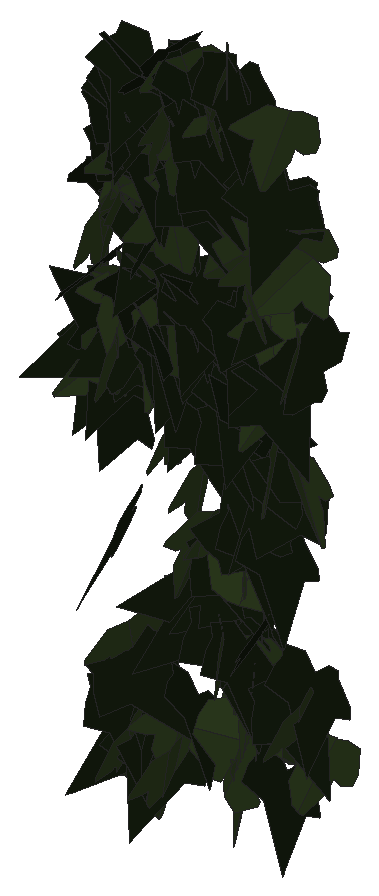
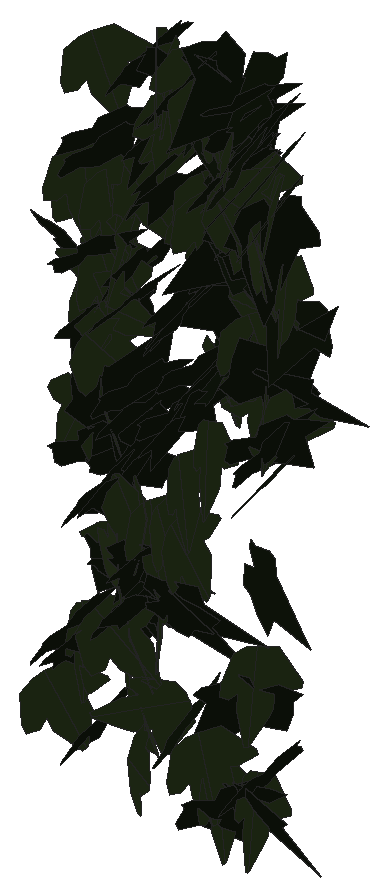
# SketchUp Ruby script. Lengths in inches.
U = 1.inch
M = Sketchup.active_model
def pt(a) = Geom::Point3d.new(a.map { |v| v * U })
def face(e, loops, mat)
  f = e.add_face(loops[0].map { |a| pt(a) })
  loops[1..].each { |l| e.add_face(l.map { |a| pt(a) }).erase! }
  f.material = f.back_material = mat if mat
  f
end
# faces: each face lists its corners as indices into pts; further lists are holes
def faces(e, pts, list, mat = nil) = list.each { |f| face(e, (f[0].is_a?(Array) ? f : [f]).map { |l| l.map { |i| pts[i] } }, mat) }
# xy, xz, yz: faces in a plane at the given z, y or x. An outline is a flat list of corners, or four numbers for a rectangle; further outlines are holes
def ring(l) = l.size == 4 ? [[l[0], l[1]], [l[2], l[1]], [l[2], l[3]], [l[0], l[3]]] : l.each_slice(2).to_a
def flat(e, list, mat, &to3) = list.each { |f| face(e, (f[0].is_a?(Array) ? f : [f]).map { |l| ring(l).map { |u, v| to3.(u, v) } }, mat) }
def xy(e, z, list, mat = nil) = flat(e, list, mat) { |x, y| [x, y, z] }
def xz(e, y, list, mat = nil) = flat(e, list, mat) { |x, z| [x, y, z] }
def yz(e, x, list, mat = nil) = flat(e, list, mat) { |y, z| [x, y, z] }
def lines(e, pts, list) = list.each { |a, b| e.add_line(pt(pts[a]), pt(pts[b])) }
# prism: a flat outline (further loops are holes) pulled along v
def prism(e, loops, v, mat = nil)
  f = face(e, loops, mat); d = Geom::Vector3d.new(v.map { |x| x * U })
  f.pushpull(f.normal.samedirection?(d) ? d.length : -d.length)
end
def box(e, o, s, mat = nil) = prism(e, [[o, [o[0] + s[0], o[1], o[2]], [o[0] + s[0], o[1] + s[1], o[2]], [o[0], o[1] + s[1], o[2]]]], [0, 0, s[2]], mat)
def at(x, y, z, deg = 0) = Geom::Transformation.translation(pt([x, y, z])) * Geom::Transformation.rotation(ORIGIN, Z_AXIS, deg.degrees)
def axes(o, x, y, z) = Geom::Transformation.new([*x, 0, *y, 0, *z, 0, *pt(o).to_a, 1])
def part(name) = M.definitions.add(name)
# library, detail: a bought-in or finely detailed component or shape, given as its bounding box
def library(name, o, s) = part(name).tap { |d| box(d.entities, o, s) }
def detail(e, o, s) = box(e.add_group.entities, o, s)
def put(e, d, t, mat = nil) = e.add_instance(d, t).tap { |i| i.material = mat if mat }
def group(e, t, mat = nil) = e.add_group.tap { |g| g.transformation = t; g.material = mat if mat }.entities
root = M.entities
M.materials.add("efeu1").color = [18, 25, 13]
M.materials.add("efeu2").color = [43, 57, 29]
c1 = part("ivyleaf_9")
p = [[1.54,2.16,1.25],[1.36,2.04,1.19],[-0.21,0.99,0.68],[-0.71,1.11,0.82],[-0.85,0.86,0.67],[-0.8,0.17,0.21],
  [-0.9,-0.01,0.1],[-0.67,-0.16,-0.02],[-0.08,-0.08,-0.05],[-0.03,-0.6,-0.4],[0.65,-0.88,-0.66],[0.83,-0.6,-0.49],
  [1.29,-0.42,-0.43],[1.8125,-0.07,-0.26],[1.21,0.44,0.15]]
faces(c1.entities,p,[[0,1,2,3,4,5,6,7,8,9,10,11,12,13,14]],"efeu1")
c2 = part("ivyleaf_10")
p = [[0,0.5,-0.03],[-0.0625,2.02,-0.43],[-0.19,2.01,-0.46],[-0.54,1.05,-0.29],[-0.52,0.625,-0.18],[-0.83,0.76,-0.28],
  [-1.16,0.64,-0.33],[-1.15,0.33,-0.24],[-0.77,-0.39,0.02],[-0.3,-0.51,0.16],[0.04,-0.48,0.23],[-0.02,2.01,-0.4375],
  [-0.06,2.01,-0.43],[0.04,-0.49,0.23],[0.67,-0.49,0.14],[1.38,0.36,-0.2],[1.375,0.51,-0.24],[0.81,0.65,-0.19],
  [0.62,0.59,-0.15],[0.6,1.09,-0.28],[0.5,1.23,-0.31]]
faces(c2.entities,p,[[0,1,2,3,4,5,6,7,8,9,10],[11,12,0,13,14,15,16,17,18,19,20]],"efeu2")
put(root,c1,axes([15.86,223.1875,230.26],[0.24677,0.30074,-0.3141],[-0.1921,-0.24861,-0.38896],[-0.39013,0.31264,-0.00716]))
put(root,c1,axes([15.21,223.49,229.13],[-0.44051,-0.07875,0.22305],[-0.21292,-0.07339,-0.44641],[0.10305,-0.48827,0.03112]))
put(root,c2,axes([17.25,223.3,223.22],[0.3938,-0.27521,-0.13851],[0.11664,-0.07489,0.4804],[-0.28517,-0.41067,0.00522]))
put(root,c1,axes([17.35,223.44,225.26],[0.03816,-0.49443,-0.06386],[-0.01235,0.06309,-0.49585],[0.49839,0.03942,-0.0074]))
put(root,c2,axes([17.53,223.3125,231.32],[-0.30315,-0.07469,0.39054],[-0.37436,-0.11188,-0.31199],[0.13399,-0.48157,0.01191]))
put(root,c2,axes([17.13,223.14,225.3125],[0.25962,-0.35479,-0.23817],[-0.02245,0.26697,-0.42217],[0.42672,0.2299,0.12269]))
put(root,c1,axes([15.59,223.49,232.23],[0.11472,-0.48546,0.03423],[0.00403,-0.03422,-0.49881],[0.48664,0.11473,-0.00394]))
put(root,c1,axes([17.7,223.23,226.99],[-0.45124,-0.18685,0.10709],[0.11532,0.00032,0.48652],[-0.18188,0.46378,0.0428]))
put(root,c2,axes([15.62,223.3,232.11],[-0.28032,-0.41388,0.01113],[-0.00701,-0.0087,-0.49988],[0.41397,-0.28041,-0.00092]))
put(root,c2,axes([15.84,223.23,230.14],[0.04541,0.05609,-0.49476],[-0.48178,0.13048,-0.02942],[0.12581,0.4794,0.0659]))
put(root,c1,axes([17.85,223.28,225.91],[-0.26617,0.38506,-0.17573],[0.10204,-0.14309,-0.4681],[-0.41078,-0.28505,-0.00241]))
put(root,c2,axes([15.21,223.46,231.27],[0.24763,-0.41301,0.13453],[0.05903,-0.12142,-0.48143],[0.43034,0.25432,-0.01137]))
put(root,c2,axes([17.3,223.51,224.67],[0.31176,-0.23758,0.31042],[0.24588,-0.18948,-0.39197],[0.30389,0.39705,-0.00131]))
put(root,c1,axes([18.74,223.23,229.96],[-0.3068,0.24738,0.3077],[-0.28197,0.13547,-0.39005],[-0.27635,-0.41286,0.05638]))
put(root,c2,axes([14.95,223.625,228.75],[0.10418,0.16205,-0.46139],[-0.21361,-0.40928,-0.19198],[-0.4399,0.23712,-0.01604]))
put(root,c1,axes([16.83,223.35,232.36],[0.12613,-0.43747,-0.20666],[-0.01007,0.21114,-0.45312],[0.48373,0.11847,0.04445]))
put(root,c2,axes([16.16,223.43,231.67],[-0.31513,-0.34515,0.17768],[-0.10555,-0.14404,-0.46702],[0.37357,-0.33185,0.01792]))
put(root,c1,axes([15.26,223.67,232.83],[-0.01589,-0.45199,0.21319],[-0.00074,-0.21328,-0.45223],[0.49975,-0.01469,0.00611]))
put(root,c2,axes([16.0625,223.44,232.81],[0.11558,-0.48244,0.06237],[0.00528,-0.06286,-0.496],[0.48643,0.11532,-0.00944]))
put(root,c1,axes([16.43,223.7,229.87],[-0.06282,-0.44757,0.21386],[0.01955,-0.21763,-0.44973],[0.49565,-0.04814,0.04484]))
put(root,c1,axes([15.47,223.64,232.97],[-0.16707,-0.46805,0.05495],[-0.00932,-0.05501,-0.49688],[0.47117,-0.16705,0.00966]))
put(root,c2,axes([18.2,223.35,229.95],[0.26547,-0.4145,-0.08784],[-0.00901,0.09811,-0.4902],[0.42361,0.26185,0.04463]))
put(root,c1,axes([17.79,223.59,226.87],[0.05152,-0.49494,0.04876],[-0.00165,-0.04919,-0.49757],[0.49734,0.05111,-0.0067]))
put(root,c2,axes([18.29,223.3,224.55],[0.03,-0.47542,-0.1519],[-0.00786,0.15171,-0.47636],[0.49904,0.03097,0.00163]))
put(root,c2,axes([15.48,223.3,224.87],[-0.17216,-0.45368,-0.12057],[0.02813,0.11822,-0.48501],[0.46858,-0.17378,-0.01518]))
put(root,c1,axes([17.84,223.66,232.11],[-0.19505,-0.45699,0.05581],[-0.00161,-0.05994,-0.49639],[0.46039,-0.19382,0.02191]))
put(root,c2,axes([15.37,223.49,229.89],[-0.32684,-0.34111,0.16377],[-0.05059,-0.17506,-0.46561],[0.37499,-0.32093,0.07992]))
put(root,c1,axes([15.02,222.98,230.23],[0.10792,0.42864,0.23371],[-0.03637,0.24575,-0.43392],[-0.48686,0.07665,0.08422]))
put(root,c1,axes([17.84,223.64,223.38],[0.05191,-0.48216,0.12178],[-0.00176,-0.12261,-0.48473],[0.4973,0.04989,-0.01443]))
put(root,c1,axes([15.3,223.51,226.43],[-0.34724,0.20864,-0.29308],[0.22682,-0.18921,-0.40343],[-0.27925,-0.41312,0.03675]))
put(root,c2,axes([17.75,223.42,231.16],[-0.17923,-0.46553,0.03403],[-0.01528,-0.03058,-0.49883],[0.46652,-0.17985,-0.00326]))
put(root,c2,axes([16.66,223.1,232.64],[-0.11534,-0.27013,-0.40463],[0.19892,0.35331,-0.29257],[0.44399,-0.22847,0.02596]))
put(root,c1,axes([15.83,223.41,230.98],[-0.36766,0.30773,-0.14188],[0.0951,-0.10723,-0.47902],[-0.32524,-0.37921,0.02032]))
put(root,c1,axes([17.04,223.51,225.42],[-0.04802,-0.46925,-0.16583],[0.04016,0.1624,-0.47118],[0.49607,-0.05858,0.02209]))
put(root,c1,axes([17.48,223.58,227.08],[0.05363,-0.49662,-0.02218],[-0.00311,0.02197,-0.49951],[0.49711,0.05371,-0.00073]))
put(root,c1,axes([16.58,223.42,232.98],[0.18734,-0.43311,-0.1653],[0.00438,0.17994,-0.46648],[0.46356,0.17333,0.07121]))
put(root,c1,axes([17.29,223.31,230.3],[0.22014,-0.34812,-0.28346],[-0.07722,0.28164,-0.40585],[0.44224,0.22246,0.07024]))
put(root,c2,axes([16.16,223.375,231.28],[-0.33531,-0.36449,-0.06867],[0.07402,0.02496,-0.49386],[0.36344,-0.34136,0.03722]))
put(root,c1,axes([15.51,223.72,233.31],[-0.22317,-0.43975,0.08259],[0.01864,-0.10135,-0.48927],[0.44705,-0.2153,0.06163]))
put(root,c2,axes([15.86,223.49,229.29],[0.46364,-0.18186,0.04437],[0.03985,-0.01991,-0.49801],[0.1829,0.46533,-0.00397]))
put(root,c1,axes([15.78,223.74,230.86],[-0.26233,-0.40787,0.12178],[-0.04372,-0.11647,-0.48428],[0.42341,-0.26472,0.02545]))
put(root,c1,axes([15.5,223.33,224.49],[0.00889,-0.2958,-0.40302],[0.13521,0.38948,-0.28288],[0.48129,-0.10396,0.08691]))
put(root,c1,axes([15.63,223.6,232.18],[0.02676,-0.49747,-0.04252],[0.01403,0.04331,-0.49792],[0.49909,0.02546,0.01627]))
put(root,c2,axes([15.36,223.5,229.1875],[-0.28977,0.20402,-0.35272],[0.28631,-0.20602,-0.35438],[-0.28993,-0.40735,0.00257]))
put(root,c2,axes([15.99,223.42,223.01],[0.00465,-0.49582,-0.06434],[-0.00297,0.06431,-0.49584],[0.49997,0.00499,-0.00235]))
put(root,c1,axes([15.07,223.65,229.21],[0.10962,0.07724,0.48168],[-0.43915,-0.19938,0.13191],[0.21245,-0.45198,0.02413]))
put(root,c2,axes([17.88,223.57,233.21],[-0.31192,-0.35447,0.16448],[-0.04207,-0.17877,-0.46505],[0.3885,-0.30396,0.0817]))
put(root,c1,axes([17.27,223.81,229.78],[-0.12009,-0.43821,0.2087],[0.02981,-0.22124,-0.4474],[0.48445,-0.09502,0.07926]))
put(root,c1,axes([16.68,223.6,225.49],[-0.49621,-0.02764,0.05486],[-0.05466,-0.00502,-0.49698],[0.02803,-0.49921,0.00196]))
put(root,c1,axes([17.75,223.48,229.39],[0.02124,-0.43309,-0.24896],[0.0132,0.24958,-0.43305],[0.49937,0.01183,0.02203]))
put(root,c2,axes([15.19,223.34,228.98],[0.1464,-0.4323,-0.20416],[0.02054,0.21901,-0.44901],[0.47765,0.12308,0.08188]))
put(root,c1,axes([15.63,223.79,229.33],[0.02375,-0.33085,0.37413],[0.13642,-0.35601,-0.32349],[0.48044,0.11745,0.07336]))
put(root,c2,axes([14.88,223.37,230.83],[0.11212,-0.45357,-0.17804],[0.04122,0.19087,-0.46029],[0.48552,0.08853,0.0802]))
put(root,c2,axes([18.15,223.52,231.125],[0.36253,0.14287,-0.31331],[-0.32168,-0.02182,-0.38216],[-0.12287,0.47866,0.0761]))
put(root,c1,axes([16.3,223.75,233.33],[0.02018,-0.49002,0.09731],[0.00339,-0.09725,-0.49044],[0.49958,0.02046,-0.0006]))
put(root,c2,axes([17.82,223.41,229.89],[0.44554,0.21775,0.06389],[-0.05854,-0.02571,0.49589],[0.21925,-0.44936,0.00258]))
put(root,c1,axes([16.27,223.76,223.92],[0.12233,-0.43677,0.21041],[0.06538,-0.20016,-0.4535],[0.48038,0.13846,0.00814]))
put(root,c2,axes([17.39,223.33,226.2],[0.40222,0.25461,-0.15297],[0.12372,0.09048,0.47593],[0.27003,-0.4207,0.00979]))
put(root,c1,axes([15.87,223.75,229.33],[0.07157,-0.48017,0.11964],[0.01452,-0.11879,-0.48547],[0.49464,0.07297,-0.00307]))
put(root,c1,axes([16.42,223.55,231.86],[0.06953,-0.46074,-0.18134],[0.055,0.18917,-0.45955],[0.49208,0.04395,0.07699]))
put(root,c2,axes([16.93,223.22,233.22],[-0.22253,0.26397,0.36166],[-0.25815,0.25434,-0.34448],[-0.36584,-0.34004,0.02309]))
put(root,c2,axes([16.88,223.34,223.83],[-0.07816,-0.12764,-0.47707],[0.4657,0.14169,-0.11421],[0.16435,-0.4622,0.09674]))
put(root,c1,axes([16.95,223.71,233.54],[0.05308,-0.49677,0.01999],[0.00139,-0.01995,-0.4996],[0.49717,0.0531,-0.00073]))
put(root,c2,axes([16.4,223.69,226.57],[0.03393,-0.46005,0.19287],[0.03089,-0.19101,-0.46104],[0.49789,0.04321,0.01546]))
put(root,c1,axes([16.08,223.8125,229.32],[-0.17918,-0.46,0.07933],[0.01217,-0.08955,-0.49177],[0.46663,-0.1743,0.04329]))
put(root,c2,axes([16.64,223.46,232.72],[-0.28671,-0.3972,-0.10015],[0.09238,0.05639,-0.48814],[0.39908,-0.29841,0.04105]))
put(root,c2,axes([17.68,223.64,230.17],[-0.14365,-0.46264,0.12379],[0.01813,-0.1344,-0.48126],[0.47858,-0.13378,0.05539]))
put(root,c1,axes([14.93,223.88,227.95],[-0.0649,-0.40738,0.28254],[0.04362,-0.28854,-0.40601],[0.49385,-0.02805,0.07299]))
put(root,c1,axes([15.2,223.5,233.45],[0.40522,-0.28286,0.07608],[0.10466,0.01853,-0.48857],[0.27357,0.41188,0.07423]))
put(root,c2,axes([17.06,223.79,223.09],[0.14308,-0.29862,0.37464],[0.25412,-0.28415,-0.32354],[0.40614,0.28299,0.07045]))
put(root,c1,axes([16.48,223.66,233.55],[-0.34415,-0.27309,-0.23871],[0.19262,0.14123,-0.43926],[0.30734,-0.3943,0.008]))
put(root,c2,axes([17.39,223.82,225.82],[0.07444,-0.25911,-0.42109],[0.16703,-0.38762,0.26804],[-0.46536,-0.18058,0.02885]))
put(root,c1,axes([16.26,223.64,232.63],[-0.43972,0.18535,-0.1493],[0.11487,-0.10941,-0.47417],[-0.20844,-0.4513,0.05363]))
put(root,c1,axes([16.61,223.51,232.05],[0.20943,-0.4047,-0.20581],[-0.03505,0.21156,-0.45168],[0.45267,0.20362,0.06025]))
put(root,c1,axes([17.96,223.58,224.62],[0.09813,-0.45117,-0.19189],[0.01714,0.19873,-0.45849],[0.48998,0.08341,0.05447]))
put(root,c2,axes([15.51,223.82,231.92],[-0.12978,-0.2891,0.38675],[-0.11233,-0.37141,-0.31533],[0.46962,-0.16873,0.03146]))
put(root,c1,axes([16,223.57,233.09],[0.35881,-0.34609,-0.03838],[-0.02774,0.02653,-0.49852],[0.34711,0.35988,-0.00017]))
put(root,c1,axes([15.06,223.69,223.61],[0.1087,-0.48477,-0.05638],[-0.0015,0.05743,-0.49669],[0.48804,0.10815,0.01103]))
put(root,c2,axes([16.99,223.77,226.72],[-0.16941,0.22803,-0.41146],[0.18439,-0.37015,-0.28105],[-0.43278,-0.24697,0.04132]))
put(root,c1,axes([17.875,223.86,227.6],[-0.35818,-0.33385,0.10122],[-0.05736,-0.08674,-0.48907],[0.34411,-0.36196,0.02384]))
put(root,c2,axes([15.125,223.36,231.96],[-0.29089,0.34506,0.21522],[-0.14504,0.15918,-0.45125],[-0.37993,-0.32496,0.00749]))
put(root,c2,axes([17.53,223.79,228.23],[0.27149,-0.28888,0.3047],[0.21672,-0.21437,-0.39634],[0.35962,0.34727,0.00881]))
put(root,c2,axes([17.63,223.86,229.07],[-0.18357,-0.31543,0.34177],[-0.0139,-0.36355,-0.34299],[0.46488,-0.13542,0.1247]))
put(root,c2,axes([15.33,223.46,223.16],[-0.00778,-0.45175,-0.21414],[0.00087,0.21416,-0.45181],[0.49994,-0.00741,-0.00255]))
put(root,c1,axes([16.36,223.68,228.39],[0.13404,-0.46899,-0.10992],[-0.00666,0.11229,-0.48718],[0.48165,0.13207,0.02386]))
put(root,c2,axes([18.06,223.61,231.48],[-0.32962,-0.37321,0.04544],[-0.02985,-0.03426,-0.49793],[0.37478,-0.33097,0.00031]))
put(root,c1,axes([15.36,223.76,232.52],[0.25717,-0.40741,0.13371],[0.08257,-0.10595,-0.48162],[0.42077,0.2698,0.01279]))
put(root,c2,axes([15.76,223.62,232.71],[-0.35355,0.31487,-0.1608],[0.08403,-0.14605,-0.47075],[-0.34342,-0.3599,0.05036]))
put(root,c1,axes([15.6875,223.85,223.06],[-0.26929,-0.42114,-0.01092],[0.00374,0.01058,-0.49987],[0.42127,-0.26931,-0.00255]))
put(root,c1,axes([16.99,223.69,228.37],[0.06031,-0.47306,-0.15024],[0.00631,0.15207,-0.47627],[0.49631,0.05555,0.02432]))
put(root,c1,axes([15.34,223.71,223.18],[-0.49579,0.06457,-0.0052],[0.00487,-0.00285,-0.49997],[-0.06459,-0.49581,0.0022]))
put(root,c2,axes([16.67,223.69,226.71],[0.10039,-0.48832,0.03824],[0.00541,-0.03793,-0.49853],[0.48979,0.1005,-0.00234]))
put(root,c1,axes([15.16,223.44,231.73],[0.2273,0.40725,-0.18023],[-0.1021,-0.1493,-0.46614],[-0.43349,0.24871,0.01529]))
put(root,c1,axes([16.26,223.66,230.28],[0.1301,-0.45127,-0.17155],[-0.00733,0.1758,-0.46802],[0.48272,0.12429,0.03913]))
put(root,c2,axes([17.59,223.73,224.93],[-0.28094,-0.20232,0.36075],[-0.30334,-0.19568,-0.34597],[0.28118,-0.41325,-0.01279]))
put(root,c1,axes([15.32,223.71,232.18],[0.21657,-0.44655,-0.06074],[0.00316,0.06889,-0.49522],[0.45065,0.21412,0.03266]))
put(root,c1,axes([18.1,223.9,224.83],[0.0081,-0.48932,0.10247],[0.00412,-0.10241,-0.48938],[0.49992,0.00878,0.00237]))
put(root,c1,axes([14.91,223.64,232.53],[0.27829,-0.39919,-0.11489],[-0.02772,0.12014,-0.48456],[0.41447,0.27607,0.04474]))
put(root,c2,axes([16.43,223.61,227.49],[0.06611,-0.48795,-0.0868],[-0.00157,0.08736,-0.49231],[0.49561,0.06537,0.01002]))
put(root,c1,axes([17.25,223.9,226.1],[-0.43068,-0.18751,0.17132],[-0.14614,-0.0929,-0.46906],[0.20774,-0.4541,0.02521]))
put(root,c2,axes([17.78,223.8,229.65],[-0.1505,-0.02069,0.47636],[-0.37965,-0.29702,-0.13285],[0.28848,-0.40169,0.07369]))
put(root,c1,axes([17.6,223.95,232.05],[-0.16455,-0.46189,0.09791],[0.0012,-0.10409,-0.48904],[0.47215,-0.16071,0.03537]))
put(root,c2,axes([16.03,223.72,223.61],[-0.23917,-0.42918,0.09274],[-0.01143,-0.09948,-0.48987],[0.43894,-0.23644,0.03777]))
put(root,c2,axes([16.07,223.51,228.08],[0.05573,-0.43751,-0.23553],[-0.03141,0.23343,-0.44105],[0.49589,0.06396,-0.00147]))
put(root,c1,axes([14.9,223.68,231.9],[0.27433,-0.40913,-0.08577],[-0.03049,0.08273,-0.49216],[0.41691,0.27526,0.02044]))
put(root,c2,axes([17.54,223.37,230.625],[-0.22344,0.31659,0.31598],[-0.18073,0.2592,-0.38749],[-0.40915,-0.28739,-0.0014]))
put(root,c1,axes([16.62,223.75,225.63],[-0.40551,0.0351,0.29039],[-0.28905,0.02794,-0.40702],[-0.0448,-0.49798,-0.00237]))
put(root,c1,axes([17.41,223.8,228.11],[0.27316,0.00482,0.41876],[-0.41754,-0.03551,0.27277],[0.03237,-0.49871,-0.01538]))
put(root,c2,axes([15.91,223.77,231.61],[-0.28617,-0.38922,0.1289],[0.00711,-0.16188,-0.47301],[0.40994,-0.2689,0.09819]))
put(root,c1,axes([14.83,224,228.5625],[-0.09371,-0.44648,0.20463],[-0.05069,-0.19842,-0.45614],[0.48852,-0.10624,-0.00807]))
put(root,c2,axes([15.46,223.87,231.43],[-0.05696,-0.04249,-0.49492],[0.359,-0.34783,-0.01145],[-0.34333,-0.35666,0.07013]))
put(root,c2,axes([18.08,223.7,227.99],[-0.40323,0.19708,-0.22039],[0.16028,-0.16748,-0.44301],[-0.24844,-0.42792,0.07189]))
put(root,c2,axes([16.85,223.68,226.72],[-0.10329,-0.48886,-0.0185],[0.00249,0.01838,-0.49966],[0.48921,-0.10331,-0.00137]))
put(root,c2,axes([16.23,223.57,233.53],[-0.3184,-0.35936,-0.13958],[0.07871,0.11662,-0.4798],[0.37739,-0.32751,-0.01769]))
put(root,c1,axes([14.89,223.97,228.75],[-0.28701,-0.40337,0.07011],[-0.02911,-0.0653,-0.49486],[0.40838,-0.28814,0.014]))
put(root,c1,axes([15.9,223.5625,229.19],[0.24989,-0.33399,-0.2757],[-0.08503,0.27427,-0.40932],[0.42465,0.25145,0.08028]))
put(root,c2,axes([18.37,223.86,223.79],[-0.28039,-0.34371,0.23074],[-0.05507,-0.24524,-0.43223],[0.4103,-0.2678,0.09967]))
put(root,c1,axes([17.75,224.05,230.5],[-0.30596,-0.35193,0.18037],[-0.04482,-0.19572,-0.45791],[0.39291,-0.29637,0.08822]))
put(root,c2,axes([15.05,223.77,231.38],[0.1605,-0.47292,0.0242],[0.00426,-0.02411,-0.4994],[0.47352,0.16052,-0.00371]))
put(root,c1,axes([15.78,223.28,233.39],[0.20782,0.35646,0.28239],[0.10768,0.26308,-0.41133],[-0.44183,0.23178,0.03258]))
put(root,c1,axes([15.33,223.45,231.375],[0.4616,0.12933,0.14212],[0.13141,0.05734,-0.479],[-0.1402,0.47957,0.01895]))
put(root,c2,axes([16.84,223.57,233.6],[0.18175,-0.40618,-0.22801],[-0.02574,0.23562,-0.44025],[0.46509,0.17177,0.06474]))
put(root,c1,axes([17,223.99,228.77],[-0.136,-0.47618,0.06898],[-0.00384,-0.07061,-0.49497],[0.48113,-0.13516,0.01555]))
put(root,c1,axes([16.76,223.74,226.35],[0.12722,-0.44939,-0.17851],[0.01655,0.18852,-0.4628],[0.48326,0.11185,0.06285]))
put(root,c1,axes([16.29,224.03,228.64],[-0.21765,-0.43639,0.11039],[-0.01304,-0.11645,-0.48607],[0.44995,-0.21447,0.03931]))
put(root,c1,axes([16.2,223.96,230.11],[0.07697,-0.48203,0.10826],[0.01398,-0.10739,-0.48813],[0.49384,0.07817,-0.00306]))
